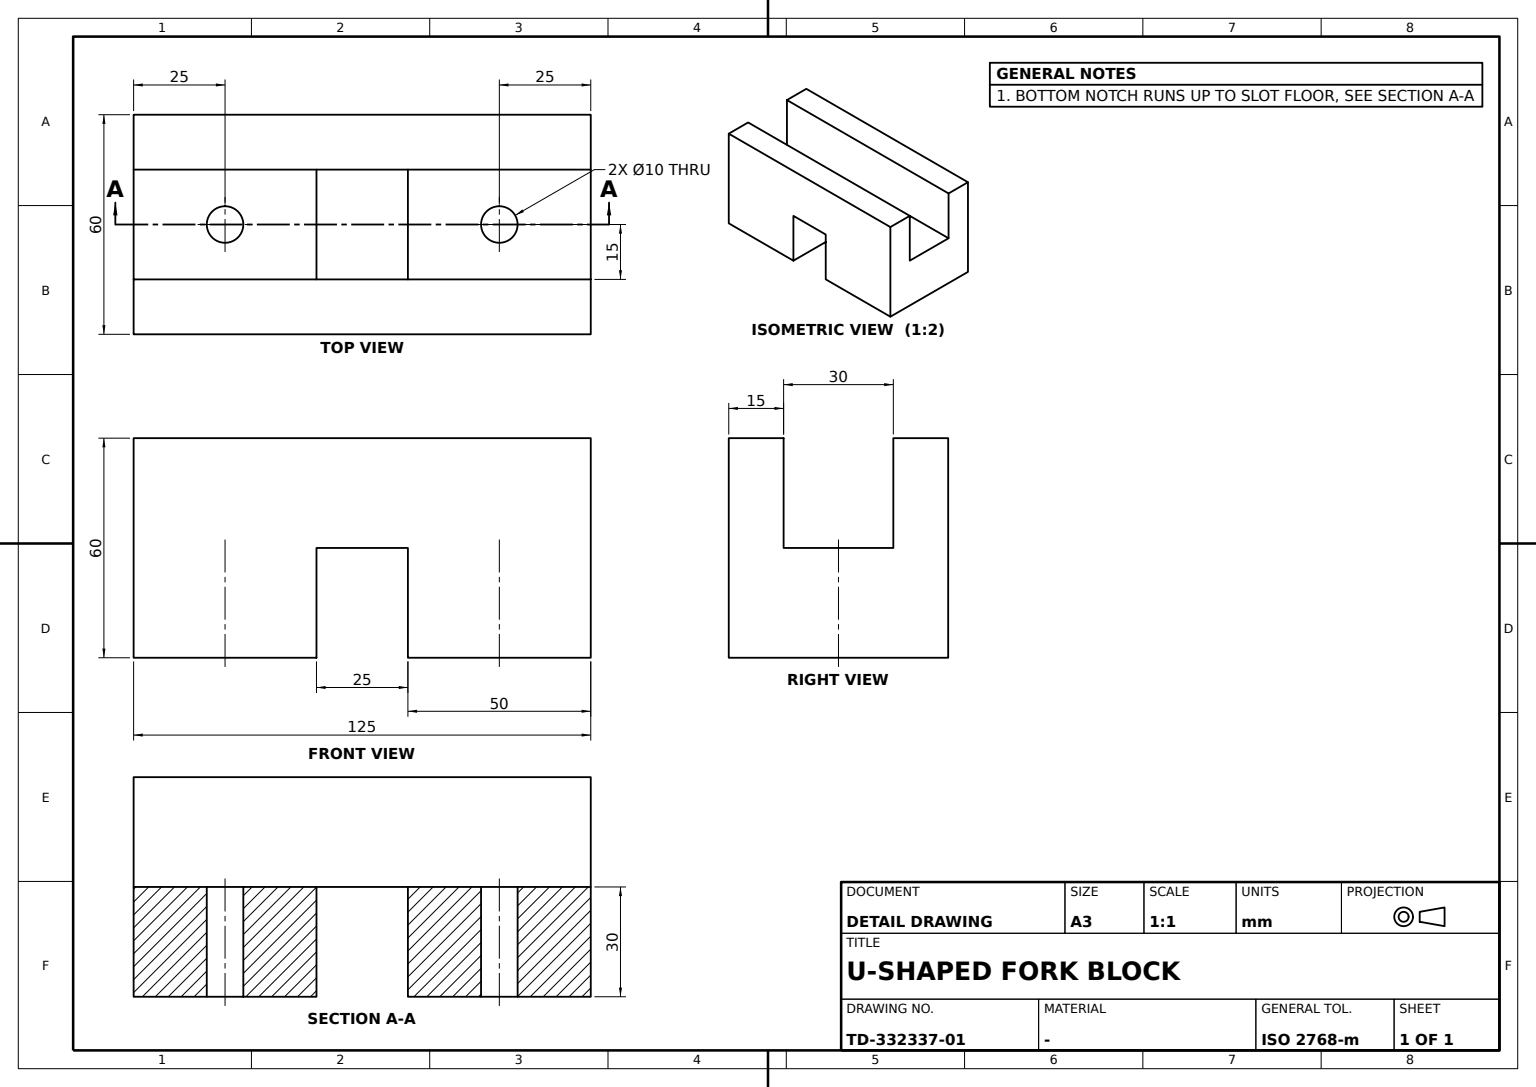
ISO-10303-21;
HEADER;
FILE_DESCRIPTION((''),'2;1');
FILE_NAME('','',(''),(''),'','','');
FILE_SCHEMA(('AUTOMOTIVE_DESIGN'));
ENDSEC;
DATA;
#1=APPLICATION_CONTEXT('');
#2=PRODUCT_CONTEXT('',#1,'mechanical');
#3=PRODUCT('','','',(#2));
#4=PRODUCT_DEFINITION_FORMATION('','',#3);
#5=PRODUCT_DEFINITION_CONTEXT('',#1,'design');
#6=PRODUCT_DEFINITION('','',#4,#5);
#7=PRODUCT_DEFINITION_SHAPE('','',#6);
#8=(LENGTH_UNIT()NAMED_UNIT(*)SI_UNIT(.MILLI.,.METRE.));
#9=(NAMED_UNIT(*)PLANE_ANGLE_UNIT()SI_UNIT($,.RADIAN.));
#10=(NAMED_UNIT(*)SI_UNIT($,.STERADIAN.)SOLID_ANGLE_UNIT());
#11=UNCERTAINTY_MEASURE_WITH_UNIT(LENGTH_MEASURE(1.E-05),#8,'distance_accuracy_value','');
#12=(GEOMETRIC_REPRESENTATION_CONTEXT(3)GLOBAL_UNCERTAINTY_ASSIGNED_CONTEXT((#11))GLOBAL_UNIT_ASSIGNED_CONTEXT((#8,#9,#10))REPRESENTATION_CONTEXT('',''));
#13=CARTESIAN_POINT('',(15.,62.5,60.));
#14=VERTEX_POINT('',#13);
#15=CARTESIAN_POINT('',(15.,62.5,30.));
#16=VERTEX_POINT('',#15);
#17=CARTESIAN_POINT('',(15.,62.5,45.));
#18=DIRECTION('',(0.,0.,-1.));
#19=VECTOR('',#18,1000.);
#20=LINE('',#17,#19);
#21=EDGE_CURVE('',#14,#16,#20,.T.);
#22=ORIENTED_EDGE('',*,*,#21,.T.);
#23=CARTESIAN_POINT('',(15.,12.5,30.));
#24=VERTEX_POINT('',#23);
#25=CARTESIAN_POINT('',(15.,37.5,30.));
#26=DIRECTION('',(0.,-1.,0.));
#27=VECTOR('',#26,1000.);
#28=LINE('',#25,#27);
#29=EDGE_CURVE('',#16,#24,#28,.T.);
#30=ORIENTED_EDGE('',*,*,#29,.T.);
#31=CARTESIAN_POINT('',(15.,-12.5,30.));
#32=VERTEX_POINT('',#31);
#33=CARTESIAN_POINT('',(15.,0.,30.));
#34=LINE('',#33,#27);
#35=EDGE_CURVE('',#24,#32,#34,.T.);
#36=ORIENTED_EDGE('',*,*,#35,.T.);
#37=CARTESIAN_POINT('',(15.,-62.5,30.));
#38=VERTEX_POINT('',#37);
#39=CARTESIAN_POINT('',(15.,-37.5,30.));
#40=LINE('',#39,#27);
#41=EDGE_CURVE('',#32,#38,#40,.T.);
#42=ORIENTED_EDGE('',*,*,#41,.T.);
#43=CARTESIAN_POINT('',(15.,-62.5,60.));
#44=VERTEX_POINT('',#43);
#45=CARTESIAN_POINT('',(15.,-62.5,45.));
#46=DIRECTION('',(0.,0.,1.));
#47=VECTOR('',#46,1000.);
#48=LINE('',#45,#47);
#49=EDGE_CURVE('',#38,#44,#48,.T.);
#50=ORIENTED_EDGE('',*,*,#49,.T.);
#51=CARTESIAN_POINT('',(15.,0.,60.));
#52=LINE('',#51,#27);
#53=EDGE_CURVE('',#14,#44,#52,.T.);
#54=ORIENTED_EDGE('',*,*,#53,.F.);
#55=EDGE_LOOP('',(#22,#30,#36,#42,#50,#54));
#56=FACE_OUTER_BOUND('',#55,.T.);
#57=CARTESIAN_POINT('',(15.,62.5,72.228943));
#58=DIRECTION('',(-1.,0.,0.));
#59=AXIS2_PLACEMENT_3D('',#57,#58,#18);
#60=PLANE('',#59);
#61=ADVANCED_FACE('',(#56),#60,.T.);
#62=CARTESIAN_POINT('',(5.,37.5,30.));
#63=VERTEX_POINT('',#62);
#64=CARTESIAN_POINT('',(5.,37.5,0.));
#65=VERTEX_POINT('',#64);
#66=CARTESIAN_POINT('',(5.,37.5,14.34));
#67=LINE('',#66,#19);
#68=EDGE_CURVE('',#63,#65,#67,.T.);
#69=ORIENTED_EDGE('',*,*,#68,.T.);
#70=CARTESIAN_POINT('',(-5.,37.5,0.));
#71=VERTEX_POINT('',#70);
#72=CARTESIAN_POINT('',(0.,37.5,0.));
#73=DIRECTION('',(0.,1.,0.));
#74=AXIS2_PLACEMENT_3D('',#72,#18,#73);
#75=CIRCLE('',#74,5.);
#76=EDGE_CURVE('',#65,#71,#75,.T.);
#77=ORIENTED_EDGE('',*,*,#76,.T.);
#78=CARTESIAN_POINT('',(-5.,37.5,30.));
#79=VERTEX_POINT('',#78);
#80=CARTESIAN_POINT('',(-5.,37.5,14.34));
#81=LINE('',#80,#19);
#82=EDGE_CURVE('',#79,#71,#81,.T.);
#83=ORIENTED_EDGE('',*,*,#82,.F.);
#84=CARTESIAN_POINT('',(0.,37.5,30.));
#85=DIRECTION('',(1.,0.,0.));
#86=AXIS2_PLACEMENT_3D('',#84,#46,#85);
#87=CIRCLE('',#86,5.);
#88=EDGE_CURVE('',#79,#63,#87,.T.);
#89=ORIENTED_EDGE('',*,*,#88,.T.);
#90=EDGE_LOOP('',(#69,#77,#83,#89));
#91=FACE_OUTER_BOUND('',#90,.T.);
#92=CARTESIAN_POINT('',(0.,37.5,14.34));
#93=AXIS2_PLACEMENT_3D('',#92,#18,#85);
#94=CYLINDRICAL_SURFACE('',#93,5.);
#95=ADVANCED_FACE('',(#91),#94,.F.);
#96=CARTESIAN_POINT('',(-30.,-62.5,60.));
#97=VERTEX_POINT('',#96);
#98=CARTESIAN_POINT('',(-30.,-62.5,0.));
#99=VERTEX_POINT('',#98);
#100=CARTESIAN_POINT('',(-30.,-62.5,30.));
#101=LINE('',#100,#19);
#102=EDGE_CURVE('',#97,#99,#101,.T.);
#103=ORIENTED_EDGE('',*,*,#102,.T.);
#104=CARTESIAN_POINT('',(30.,-62.5,0.));
#105=VERTEX_POINT('',#104);
#106=CARTESIAN_POINT('',(0.,-62.5,0.));
#107=VECTOR('',#85,1000.);
#108=LINE('',#106,#107);
#109=EDGE_CURVE('',#99,#105,#108,.T.);
#110=ORIENTED_EDGE('',*,*,#109,.T.);
#111=CARTESIAN_POINT('',(30.,-62.5,60.));
#112=VERTEX_POINT('',#111);
#113=CARTESIAN_POINT('',(30.,-62.5,30.));
#114=LINE('',#113,#19);
#115=EDGE_CURVE('',#112,#105,#114,.T.);
#116=ORIENTED_EDGE('',*,*,#115,.F.);
#117=CARTESIAN_POINT('',(22.5,-62.5,60.));
#118=LINE('',#117,#107);
#119=EDGE_CURVE('',#44,#112,#118,.T.);
#120=ORIENTED_EDGE('',*,*,#119,.F.);
#121=ORIENTED_EDGE('',*,*,#49,.F.);
#122=CARTESIAN_POINT('',(-15.,-62.5,30.));
#123=VERTEX_POINT('',#122);
#124=CARTESIAN_POINT('',(0.,-62.5,30.));
#125=VECTOR('',#58,1000.);
#126=LINE('',#124,#125);
#127=EDGE_CURVE('',#38,#123,#126,.T.);
#128=ORIENTED_EDGE('',*,*,#127,.T.);
#129=CARTESIAN_POINT('',(-15.,-62.5,60.));
#130=VERTEX_POINT('',#129);
#131=CARTESIAN_POINT('',(-15.,-62.5,45.));
#132=LINE('',#131,#47);
#133=EDGE_CURVE('',#123,#130,#132,.T.);
#134=ORIENTED_EDGE('',*,*,#133,.T.);
#135=CARTESIAN_POINT('',(-22.5,-62.5,60.));
#136=LINE('',#135,#107);
#137=EDGE_CURVE('',#97,#130,#136,.T.);
#138=ORIENTED_EDGE('',*,*,#137,.F.);
#139=EDGE_LOOP('',(#103,#110,#116,#120,#121,#128,#134,#138));
#140=FACE_OUTER_BOUND('',#139,.T.);
#141=AXIS2_PLACEMENT_3D('',#106,#73,#46);
#142=PLANE('',#141);
#143=ADVANCED_FACE('',(#140),#142,.F.);
#144=ORIENTED_EDGE('',*,*,#88,.F.);
#145=EDGE_CURVE('',#63,#79,#87,.T.);
#146=ORIENTED_EDGE('',*,*,#145,.F.);
#147=EDGE_LOOP('',(#144,#146));
#148=FACE_BOUND('',#147,.T.);
#149=ORIENTED_EDGE('',*,*,#29,.F.);
#150=CARTESIAN_POINT('',(-15.,62.5,30.));
#151=VERTEX_POINT('',#150);
#152=CARTESIAN_POINT('',(0.,62.5,30.));
#153=LINE('',#152,#125);
#154=EDGE_CURVE('',#16,#151,#153,.T.);
#155=ORIENTED_EDGE('',*,*,#154,.T.);
#156=CARTESIAN_POINT('',(-15.,12.5,30.));
#157=VERTEX_POINT('',#156);
#158=CARTESIAN_POINT('',(-15.,37.5,30.));
#159=LINE('',#158,#27);
#160=EDGE_CURVE('',#151,#157,#159,.T.);
#161=ORIENTED_EDGE('',*,*,#160,.T.);
#162=CARTESIAN_POINT('',(0.,12.5,30.));
#163=LINE('',#162,#107);
#164=EDGE_CURVE('',#157,#24,#163,.T.);
#165=ORIENTED_EDGE('',*,*,#164,.T.);
#166=EDGE_LOOP('',(#149,#155,#161,#165));
#167=FACE_OUTER_BOUND('',#166,.T.);
#168=CARTESIAN_POINT('',(0.,-12.5,30.));
#169=AXIS2_PLACEMENT_3D('',#168,#18,#73);
#170=PLANE('',#169);
#171=ADVANCED_FACE('',(#148,#167),#170,.F.);
#172=CARTESIAN_POINT('',(-30.,62.5,0.));
#173=VERTEX_POINT('',#172);
#174=CARTESIAN_POINT('',(-30.,62.5,60.));
#175=VERTEX_POINT('',#174);
#176=CARTESIAN_POINT('',(-30.,62.5,30.));
#177=LINE('',#176,#47);
#178=EDGE_CURVE('',#173,#175,#177,.T.);
#179=ORIENTED_EDGE('',*,*,#178,.F.);
#180=CARTESIAN_POINT('',(-30.,12.5,0.));
#181=VERTEX_POINT('',#180);
#182=CARTESIAN_POINT('',(-30.,37.5,0.));
#183=VECTOR('',#73,1000.);
#184=LINE('',#182,#183);
#185=EDGE_CURVE('',#181,#173,#184,.T.);
#186=ORIENTED_EDGE('',*,*,#185,.F.);
#187=CARTESIAN_POINT('',(-30.,12.5,30.));
#188=VERTEX_POINT('',#187);
#189=CARTESIAN_POINT('',(-30.,12.5,15.));
#190=LINE('',#189,#19);
#191=EDGE_CURVE('',#188,#181,#190,.T.);
#192=ORIENTED_EDGE('',*,*,#191,.F.);
#193=CARTESIAN_POINT('',(-30.,-12.5,30.));
#194=VERTEX_POINT('',#193);
#195=CARTESIAN_POINT('',(-30.,0.,30.));
#196=LINE('',#195,#183);
#197=EDGE_CURVE('',#194,#188,#196,.T.);
#198=ORIENTED_EDGE('',*,*,#197,.F.);
#199=CARTESIAN_POINT('',(-30.,-12.5,0.));
#200=VERTEX_POINT('',#199);
#201=CARTESIAN_POINT('',(-30.,-12.5,15.));
#202=LINE('',#201,#47);
#203=EDGE_CURVE('',#200,#194,#202,.T.);
#204=ORIENTED_EDGE('',*,*,#203,.F.);
#205=CARTESIAN_POINT('',(-30.,-37.5,0.));
#206=LINE('',#205,#183);
#207=EDGE_CURVE('',#99,#200,#206,.T.);
#208=ORIENTED_EDGE('',*,*,#207,.F.);
#209=ORIENTED_EDGE('',*,*,#102,.F.);
#210=CARTESIAN_POINT('',(-30.,0.,60.));
#211=LINE('',#210,#27);
#212=EDGE_CURVE('',#175,#97,#211,.T.);
#213=ORIENTED_EDGE('',*,*,#212,.F.);
#214=EDGE_LOOP('',(#179,#186,#192,#198,#204,#208,#209,#213));
#215=FACE_OUTER_BOUND('',#214,.T.);
#216=CARTESIAN_POINT('',(-30.,0.,0.));
#217=AXIS2_PLACEMENT_3D('',#216,#85,#73);
#218=PLANE('',#217);
#219=ADVANCED_FACE('',(#215),#218,.F.);
#220=CARTESIAN_POINT('',(30.,62.5,60.));
#221=VERTEX_POINT('',#220);
#222=CARTESIAN_POINT('',(22.5,62.5,60.));
#223=LINE('',#222,#107);
#224=EDGE_CURVE('',#14,#221,#223,.T.);
#225=ORIENTED_EDGE('',*,*,#224,.T.);
#226=CARTESIAN_POINT('',(30.,62.5,0.));
#227=VERTEX_POINT('',#226);
#228=CARTESIAN_POINT('',(30.,62.5,30.));
#229=LINE('',#228,#47);
#230=EDGE_CURVE('',#227,#221,#229,.T.);
#231=ORIENTED_EDGE('',*,*,#230,.F.);
#232=CARTESIAN_POINT('',(0.,62.5,0.));
#233=LINE('',#232,#107);
#234=EDGE_CURVE('',#173,#227,#233,.T.);
#235=ORIENTED_EDGE('',*,*,#234,.F.);
#236=ORIENTED_EDGE('',*,*,#178,.T.);
#237=CARTESIAN_POINT('',(-15.,62.5,60.));
#238=VERTEX_POINT('',#237);
#239=CARTESIAN_POINT('',(-22.5,62.5,60.));
#240=LINE('',#239,#107);
#241=EDGE_CURVE('',#175,#238,#240,.T.);
#242=ORIENTED_EDGE('',*,*,#241,.T.);
#243=CARTESIAN_POINT('',(-15.,62.5,45.));
#244=LINE('',#243,#47);
#245=EDGE_CURVE('',#151,#238,#244,.T.);
#246=ORIENTED_EDGE('',*,*,#245,.F.);
#247=ORIENTED_EDGE('',*,*,#154,.F.);
#248=ORIENTED_EDGE('',*,*,#21,.F.);
#249=EDGE_LOOP('',(#225,#231,#235,#236,#242,#246,#247,#248));
#250=FACE_OUTER_BOUND('',#249,.T.);
#251=CARTESIAN_POINT('',(0.,62.5,60.));
#252=AXIS2_PLACEMENT_3D('',#251,#26,#18);
#253=PLANE('',#252);
#254=ADVANCED_FACE('',(#250),#253,.F.);
#255=ORIENTED_EDGE('',*,*,#133,.F.);
#256=CARTESIAN_POINT('',(-15.,-12.5,30.));
#257=VERTEX_POINT('',#256);
#258=CARTESIAN_POINT('',(-15.,-37.5,30.));
#259=LINE('',#258,#27);
#260=EDGE_CURVE('',#257,#123,#259,.T.);
#261=ORIENTED_EDGE('',*,*,#260,.F.);
#262=CARTESIAN_POINT('',(-15.,0.,30.));
#263=LINE('',#262,#27);
#264=EDGE_CURVE('',#157,#257,#263,.T.);
#265=ORIENTED_EDGE('',*,*,#264,.F.);
#266=ORIENTED_EDGE('',*,*,#160,.F.);
#267=ORIENTED_EDGE('',*,*,#245,.T.);
#268=CARTESIAN_POINT('',(-15.,0.,60.));
#269=LINE('',#268,#27);
#270=EDGE_CURVE('',#238,#130,#269,.T.);
#271=ORIENTED_EDGE('',*,*,#270,.T.);
#272=EDGE_LOOP('',(#255,#261,#265,#266,#267,#271));
#273=FACE_OUTER_BOUND('',#272,.T.);
#274=AXIS2_PLACEMENT_3D('',#150,#85,#46);
#275=PLANE('',#274);
#276=ADVANCED_FACE('',(#273),#275,.T.);
#277=ORIENTED_EDGE('',*,*,#145,.T.);
#278=ORIENTED_EDGE('',*,*,#82,.T.);
#279=EDGE_CURVE('',#71,#65,#75,.T.);
#280=ORIENTED_EDGE('',*,*,#279,.T.);
#281=ORIENTED_EDGE('',*,*,#68,.F.);
#282=EDGE_LOOP('',(#277,#278,#280,#281));
#283=FACE_OUTER_BOUND('',#282,.T.);
#284=ADVANCED_FACE('',(#283),#94,.F.);
#285=CARTESIAN_POINT('',(-5.,-37.5,30.));
#286=VERTEX_POINT('',#285);
#287=CARTESIAN_POINT('',(5.,-37.5,30.));
#288=VERTEX_POINT('',#287);
#289=CARTESIAN_POINT('',(0.,-37.5,30.));
#290=AXIS2_PLACEMENT_3D('',#289,#46,#85);
#291=CIRCLE('',#290,5.);
#292=EDGE_CURVE('',#286,#288,#291,.T.);
#293=ORIENTED_EDGE('',*,*,#292,.T.);
#294=CARTESIAN_POINT('',(5.,-37.5,0.));
#295=VERTEX_POINT('',#294);
#296=CARTESIAN_POINT('',(5.,-37.5,14.34));
#297=LINE('',#296,#19);
#298=EDGE_CURVE('',#288,#295,#297,.T.);
#299=ORIENTED_EDGE('',*,*,#298,.T.);
#300=CARTESIAN_POINT('',(-5.,-37.5,0.));
#301=VERTEX_POINT('',#300);
#302=CARTESIAN_POINT('',(0.,-37.5,0.));
#303=AXIS2_PLACEMENT_3D('',#302,#18,#73);
#304=CIRCLE('',#303,5.);
#305=EDGE_CURVE('',#295,#301,#304,.T.);
#306=ORIENTED_EDGE('',*,*,#305,.T.);
#307=CARTESIAN_POINT('',(-5.,-37.5,14.34));
#308=LINE('',#307,#19);
#309=EDGE_CURVE('',#286,#301,#308,.T.);
#310=ORIENTED_EDGE('',*,*,#309,.F.);
#311=EDGE_LOOP('',(#293,#299,#306,#310));
#312=FACE_OUTER_BOUND('',#311,.T.);
#313=CARTESIAN_POINT('',(0.,-37.5,14.34));
#314=AXIS2_PLACEMENT_3D('',#313,#18,#85);
#315=CYLINDRICAL_SURFACE('',#314,5.);
#316=ADVANCED_FACE('',(#312),#315,.F.);
#317=ORIENTED_EDGE('',*,*,#279,.F.);
#318=ORIENTED_EDGE('',*,*,#76,.F.);
#319=EDGE_LOOP('',(#317,#318));
#320=FACE_BOUND('',#319,.T.);
#321=ORIENTED_EDGE('',*,*,#234,.T.);
#322=CARTESIAN_POINT('',(30.,12.5,0.));
#323=VERTEX_POINT('',#322);
#324=CARTESIAN_POINT('',(30.,37.5,0.));
#325=LINE('',#324,#183);
#326=EDGE_CURVE('',#323,#227,#325,.T.);
#327=ORIENTED_EDGE('',*,*,#326,.F.);
#328=CARTESIAN_POINT('',(0.,12.5,0.));
#329=LINE('',#328,#107);
#330=EDGE_CURVE('',#181,#323,#329,.T.);
#331=ORIENTED_EDGE('',*,*,#330,.F.);
#332=ORIENTED_EDGE('',*,*,#185,.T.);
#333=EDGE_LOOP('',(#321,#327,#331,#332));
#334=FACE_OUTER_BOUND('',#333,.T.);
#335=AXIS2_PLACEMENT_3D('',#106,#18,#73);
#336=PLANE('',#335);
#337=ADVANCED_FACE('',(#320,#334),#336,.T.);
#338=ORIENTED_EDGE('',*,*,#164,.F.);
#339=CARTESIAN_POINT('',(-22.5,12.5,30.));
#340=LINE('',#339,#107);
#341=EDGE_CURVE('',#188,#157,#340,.T.);
#342=ORIENTED_EDGE('',*,*,#341,.F.);
#343=ORIENTED_EDGE('',*,*,#191,.T.);
#344=ORIENTED_EDGE('',*,*,#330,.T.);
#345=CARTESIAN_POINT('',(30.,12.5,30.));
#346=VERTEX_POINT('',#345);
#347=CARTESIAN_POINT('',(30.,12.5,15.));
#348=LINE('',#347,#19);
#349=EDGE_CURVE('',#346,#323,#348,.T.);
#350=ORIENTED_EDGE('',*,*,#349,.F.);
#351=CARTESIAN_POINT('',(22.5,12.5,30.));
#352=LINE('',#351,#107);
#353=EDGE_CURVE('',#24,#346,#352,.T.);
#354=ORIENTED_EDGE('',*,*,#353,.F.);
#355=EDGE_LOOP('',(#338,#342,#343,#344,#350,#354));
#356=FACE_OUTER_BOUND('',#355,.T.);
#357=AXIS2_PLACEMENT_3D('',#162,#26,#18);
#358=PLANE('',#357);
#359=ADVANCED_FACE('',(#356),#358,.T.);
#360=ORIENTED_EDGE('',*,*,#341,.T.);
#361=ORIENTED_EDGE('',*,*,#264,.T.);
#362=CARTESIAN_POINT('',(-22.5,-12.5,30.));
#363=LINE('',#362,#107);
#364=EDGE_CURVE('',#194,#257,#363,.T.);
#365=ORIENTED_EDGE('',*,*,#364,.F.);
#366=ORIENTED_EDGE('',*,*,#197,.T.);
#367=EDGE_LOOP('',(#360,#361,#365,#366));
#368=FACE_OUTER_BOUND('',#367,.T.);
#369=ADVANCED_FACE('',(#368),#170,.T.);
#370=LINE('',#168,#107);
#371=EDGE_CURVE('',#257,#32,#370,.T.);
#372=ORIENTED_EDGE('',*,*,#371,.T.);
#373=CARTESIAN_POINT('',(30.,-12.5,30.));
#374=VERTEX_POINT('',#373);
#375=CARTESIAN_POINT('',(22.5,-12.5,30.));
#376=LINE('',#375,#107);
#377=EDGE_CURVE('',#32,#374,#376,.T.);
#378=ORIENTED_EDGE('',*,*,#377,.T.);
#379=CARTESIAN_POINT('',(30.,-12.5,0.));
#380=VERTEX_POINT('',#379);
#381=CARTESIAN_POINT('',(30.,-12.5,15.));
#382=LINE('',#381,#47);
#383=EDGE_CURVE('',#380,#374,#382,.T.);
#384=ORIENTED_EDGE('',*,*,#383,.F.);
#385=CARTESIAN_POINT('',(0.,-12.5,0.));
#386=LINE('',#385,#107);
#387=EDGE_CURVE('',#200,#380,#386,.T.);
#388=ORIENTED_EDGE('',*,*,#387,.F.);
#389=ORIENTED_EDGE('',*,*,#203,.T.);
#390=ORIENTED_EDGE('',*,*,#364,.T.);
#391=EDGE_LOOP('',(#372,#378,#384,#388,#389,#390));
#392=FACE_OUTER_BOUND('',#391,.T.);
#393=AXIS2_PLACEMENT_3D('',#385,#73,#46);
#394=PLANE('',#393);
#395=ADVANCED_FACE('',(#392),#394,.T.);
#396=ORIENTED_EDGE('',*,*,#115,.T.);
#397=CARTESIAN_POINT('',(30.,-37.5,0.));
#398=LINE('',#397,#183);
#399=EDGE_CURVE('',#105,#380,#398,.T.);
#400=ORIENTED_EDGE('',*,*,#399,.T.);
#401=ORIENTED_EDGE('',*,*,#383,.T.);
#402=CARTESIAN_POINT('',(30.,0.,30.));
#403=LINE('',#402,#183);
#404=EDGE_CURVE('',#374,#346,#403,.T.);
#405=ORIENTED_EDGE('',*,*,#404,.T.);
#406=ORIENTED_EDGE('',*,*,#349,.T.);
#407=ORIENTED_EDGE('',*,*,#326,.T.);
#408=ORIENTED_EDGE('',*,*,#230,.T.);
#409=CARTESIAN_POINT('',(30.,0.,60.));
#410=LINE('',#409,#27);
#411=EDGE_CURVE('',#221,#112,#410,.T.);
#412=ORIENTED_EDGE('',*,*,#411,.T.);
#413=EDGE_LOOP('',(#396,#400,#401,#405,#406,#407,#408,#412));
#414=FACE_OUTER_BOUND('',#413,.T.);
#415=CARTESIAN_POINT('',(30.,0.,0.));
#416=AXIS2_PLACEMENT_3D('',#415,#85,#73);
#417=PLANE('',#416);
#418=ADVANCED_FACE('',(#414),#417,.T.);
#419=ORIENTED_EDGE('',*,*,#292,.F.);
#420=EDGE_CURVE('',#288,#286,#291,.T.);
#421=ORIENTED_EDGE('',*,*,#420,.F.);
#422=EDGE_LOOP('',(#419,#421));
#423=FACE_BOUND('',#422,.T.);
#424=ORIENTED_EDGE('',*,*,#260,.T.);
#425=ORIENTED_EDGE('',*,*,#127,.F.);
#426=ORIENTED_EDGE('',*,*,#41,.F.);
#427=ORIENTED_EDGE('',*,*,#371,.F.);
#428=EDGE_LOOP('',(#424,#425,#426,#427));
#429=FACE_OUTER_BOUND('',#428,.T.);
#430=ADVANCED_FACE('',(#423,#429),#170,.F.);
#431=ORIENTED_EDGE('',*,*,#270,.F.);
#432=ORIENTED_EDGE('',*,*,#241,.F.);
#433=ORIENTED_EDGE('',*,*,#212,.T.);
#434=ORIENTED_EDGE('',*,*,#137,.T.);
#435=EDGE_LOOP('',(#431,#432,#433,#434));
#436=FACE_OUTER_BOUND('',#435,.T.);
#437=CARTESIAN_POINT('',(0.,-62.5,60.));
#438=AXIS2_PLACEMENT_3D('',#437,#18,#73);
#439=PLANE('',#438);
#440=ADVANCED_FACE('',(#436),#439,.F.);
#441=ORIENTED_EDGE('',*,*,#305,.F.);
#442=EDGE_CURVE('',#301,#295,#304,.T.);
#443=ORIENTED_EDGE('',*,*,#442,.F.);
#444=EDGE_LOOP('',(#441,#443));
#445=FACE_BOUND('',#444,.T.);
#446=ORIENTED_EDGE('',*,*,#109,.F.);
#447=ORIENTED_EDGE('',*,*,#207,.T.);
#448=ORIENTED_EDGE('',*,*,#387,.T.);
#449=ORIENTED_EDGE('',*,*,#399,.F.);
#450=EDGE_LOOP('',(#446,#447,#448,#449));
#451=FACE_OUTER_BOUND('',#450,.T.);
#452=ADVANCED_FACE('',(#445,#451),#336,.T.);
#453=ORIENTED_EDGE('',*,*,#442,.T.);
#454=ORIENTED_EDGE('',*,*,#298,.F.);
#455=ORIENTED_EDGE('',*,*,#420,.T.);
#456=ORIENTED_EDGE('',*,*,#309,.T.);
#457=EDGE_LOOP('',(#453,#454,#455,#456));
#458=FACE_OUTER_BOUND('',#457,.T.);
#459=ADVANCED_FACE('',(#458),#315,.F.);
#460=ORIENTED_EDGE('',*,*,#224,.F.);
#461=ORIENTED_EDGE('',*,*,#53,.T.);
#462=ORIENTED_EDGE('',*,*,#119,.T.);
#463=ORIENTED_EDGE('',*,*,#411,.F.);
#464=EDGE_LOOP('',(#460,#461,#462,#463));
#465=FACE_OUTER_BOUND('',#464,.T.);
#466=ADVANCED_FACE('',(#465),#439,.F.);
#467=ORIENTED_EDGE('',*,*,#377,.F.);
#468=ORIENTED_EDGE('',*,*,#35,.F.);
#469=ORIENTED_EDGE('',*,*,#353,.T.);
#470=ORIENTED_EDGE('',*,*,#404,.F.);
#471=EDGE_LOOP('',(#467,#468,#469,#470));
#472=FACE_OUTER_BOUND('',#471,.T.);
#473=ADVANCED_FACE('',(#472),#170,.T.);
#474=CLOSED_SHELL('',(#61,#95,#143,#171,#219,#254,#276,#284,#316,#337,#359,#369,#395,#418,#430,#440,#452,#459,#466,#473));
#475=MANIFOLD_SOLID_BREP('',#474);
#476=ADVANCED_BREP_SHAPE_REPRESENTATION('',(#475),#12);
#477=SHAPE_DEFINITION_REPRESENTATION(#7,#476);
ENDSEC;
END-ISO-10303-21;
